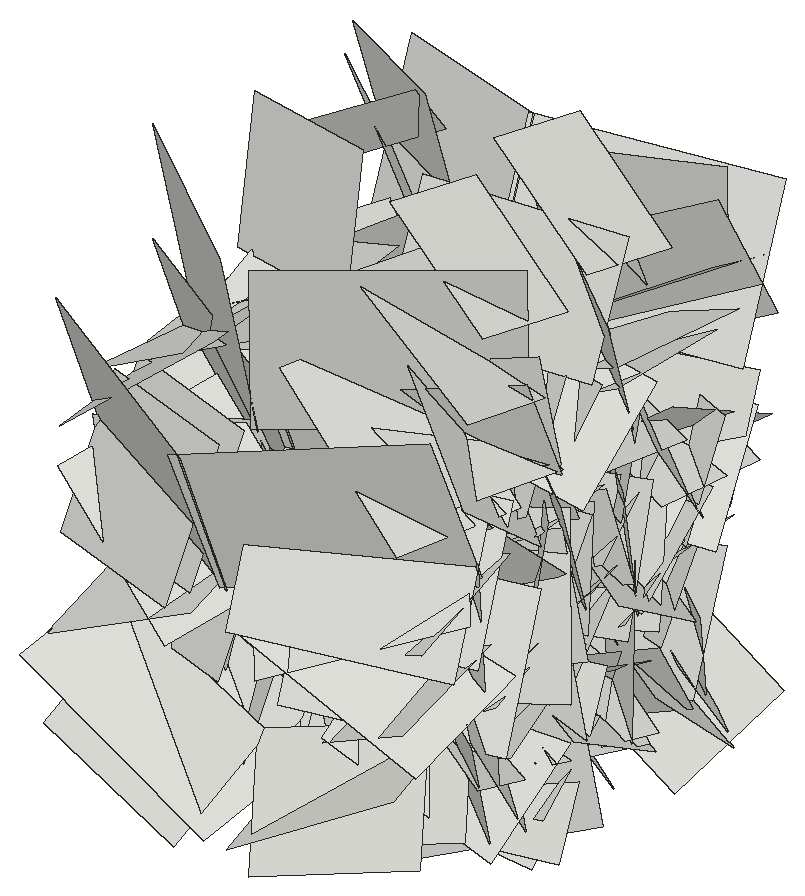
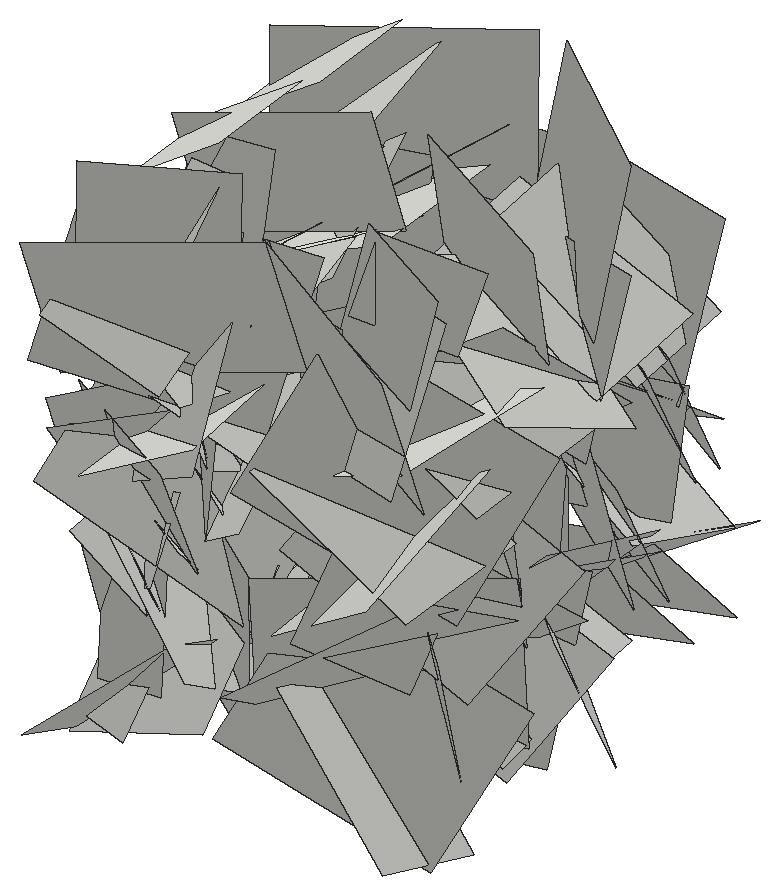
# SketchUp Ruby script. Lengths in inches.
U = 1.inch
M = Sketchup.active_model
def pt(a) = Geom::Point3d.new(a.map { |v| v * U })
def face(e, loops, mat)
  f = e.add_face(loops[0].map { |a| pt(a) })
  loops[1..].each { |l| e.add_face(l.map { |a| pt(a) }).erase! }
  f.material = f.back_material = mat if mat
  f
end
# faces: each face lists its corners as indices into pts; further lists are holes
def faces(e, pts, list, mat = nil) = list.each { |f| face(e, (f[0].is_a?(Array) ? f : [f]).map { |l| l.map { |i| pts[i] } }, mat) }
# xy, xz, yz: faces in a plane at the given z, y or x. An outline is a flat list of corners, or four numbers for a rectangle; further outlines are holes
def ring(l) = l.size == 4 ? [[l[0], l[1]], [l[2], l[1]], [l[2], l[3]], [l[0], l[3]]] : l.each_slice(2).to_a
def flat(e, list, mat, &to3) = list.each { |f| face(e, (f[0].is_a?(Array) ? f : [f]).map { |l| ring(l).map { |u, v| to3.(u, v) } }, mat) }
def xy(e, z, list, mat = nil) = flat(e, list, mat) { |x, y| [x, y, z] }
def xz(e, y, list, mat = nil) = flat(e, list, mat) { |x, z| [x, y, z] }
def yz(e, x, list, mat = nil) = flat(e, list, mat) { |y, z| [x, y, z] }
def lines(e, pts, list) = list.each { |a, b| e.add_line(pt(pts[a]), pt(pts[b])) }
# prism: a flat outline (further loops are holes) pulled along v
def prism(e, loops, v, mat = nil)
  f = face(e, loops, mat); d = Geom::Vector3d.new(v.map { |x| x * U })
  f.pushpull(f.normal.samedirection?(d) ? d.length : -d.length)
end
def box(e, o, s, mat = nil) = prism(e, [[o, [o[0] + s[0], o[1], o[2]], [o[0] + s[0], o[1] + s[1], o[2]], [o[0], o[1] + s[1], o[2]]]], [0, 0, s[2]], mat)
def at(x, y, z, deg = 0) = Geom::Transformation.translation(pt([x, y, z])) * Geom::Transformation.rotation(ORIGIN, Z_AXIS, deg.degrees)
def axes(o, x, y, z) = Geom::Transformation.new([*x, 0, *y, 0, *z, 0, *pt(o).to_a, 1])
def part(name) = M.definitions.add(name)
# library, detail: a bought-in or finely detailed component or shape, given as its bounding box
def library(name, o, s) = part(name).tap { |d| box(d.entities, o, s) }
def detail(e, o, s) = box(e.add_group.entities, o, s)
def put(e, d, t, mat = nil) = e.add_instance(d, t).tap { |i| i.material = mat if mat }
def group(e, t, mat = nil) = e.add_group.tap { |g| g.transformation = t; g.material = mat if mat }.entities
root = M.entities
c1 = part("Component\#6")
p = [[0.01,0,0],[0,3.24,4.54],[4.32,3.24,4.54],[4.33,0,0]]
faces(c1.entities,p,[[0,1,2,3]])
put(root,c1,axes([400.91,124,36.29],[-0.02149,0.52903,-1.24729],[0.2007,-1.23408,-0.5265],[1.42204,0.18216,0.05546]))
put(root,c1,axes([414.68,124,36.29],[0.02149,0.52903,-1.24729],[-0.2007,-1.23408,-0.5265],[-1.42204,0.18216,0.05546]))
put(root,c1,axes([400.85,123.49,22.43],[0.36857,0.54861,0.76203],[0.54406,0.56941,-0.64413],[0.83345,-0.61431,0.08349]))
put(root,c1,axes([414.74,123.49,22.43],[-0.36857,0.54861,0.76203],[-0.54406,0.56941,-0.64413],[-0.83345,-0.61431,0.08349]))
put(root,c1,axes([400.91,126.73,32.74],[-0.07983,-0.47542,-1.06148],[0.1788,-1.05692,0.46141],[1.21984,0.1238,-0.1371]))
put(root,c1,axes([414.68,126.73,32.74],[0.07983,-0.47542,-1.06148],[-0.1788,-1.05692,0.46141],[-1.21984,0.1238,-0.1371]))
put(root,c1,axes([400.91,122.33,25.2],[0.14417,1.26196,0.33106],[0.05821,0.32703,-1.26913],[1.38172,-0.14545,0.01892]))
put(root,c1,axes([414.68,122.33,25.2],[-0.14417,1.26196,0.33106],[-0.05821,0.32703,-1.26913],[-1.38172,-0.14545,0.01892]))
put(root,c1,axes([400.91,127.85,32.74],[-0.07983,-0.47542,-1.06148],[0.1788,-1.05692,0.46141],[1.21984,0.1238,-0.1371]))
put(root,c1,axes([414.68,127.85,32.74],[0.07983,-0.47542,-1.06148],[-0.1788,-1.05692,0.46141],[-1.21984,0.1238,-0.1371]))
put(root,c1,axes([400.91,128.39,27.01],[0.01413,-1.13969,-0.35832],[0.11214,-0.35581,1.13564],[1.2614,0.04439,-0.09695]))
put(root,c1,axes([414.68,128.39,27.01],[-0.01413,-1.13969,-0.35832],[-0.11214,-0.35581,1.13564],[-1.2614,0.04439,-0.09695]))
put(root,c1,axes([400.2,124.93,30.08],[0.69154,0.83647,0.57299],[0.50453,0.34895,-1.05134],[0.94895,-0.79509,0.14141]))
put(root,c1,axes([415.4,124.93,30.08],[-0.69154,0.83647,0.57299],[-0.50453,0.34895,-1.05134],[-0.94895,-0.79509,0.14141]))
put(root,c1,axes([410.71,128.06,26.23],[-0.10092,-0.80547,-0.37503],[-0.00485,-0.37672,0.81027],[0.94179,-0.08825,-0.03602]))
put(root,c1,axes([400.91,128.2,32.33],[0.15852,-1.12421,0.05612],[-0.12401,0.04078,1.12872],[1.18668,0.15444,0.11046]))
put(root,c1,axes([414.68,128.2,32.33],[-0.15852,-1.12421,0.05612],[0.12401,0.04078,1.12872],[-1.18668,0.15444,0.11046]))
put(root,c1,axes([400.85,125.55,22.43],[0.36857,0.54861,0.76203],[0.54406,0.56941,-0.64413],[0.83345,-0.61431,0.08349]))
put(root,c1,axes([414.74,125.55,22.43],[-0.36857,0.54861,0.76203],[-0.54406,0.56941,-0.64413],[-0.83345,-0.61431,0.08349]))
put(root,c1,axes([410.71,129.13,29.07],[-0.11411,-0.79222,-0.47459],[-0.01099,-0.47673,0.79815],[0.97884,-0.0977,-0.04636]))
put(root,c1,axes([400.91,128.47,40.0625],[0.15368,0.21217,-1.35934],[-0.08132,-1.3635,-0.221],[1.45608,-0.09854,0.13113]))
put(root,c1,axes([414.68,128.47,40.0625],[-0.15368,0.21217,-1.35934],[0.08132,-1.3635,-0.221],[-1.45608,-0.09854,0.13113]))
put(root,c1,axes([400.91,129.14,29.25],[-0.07983,-0.47542,-1.06148],[0.1788,-1.05692,0.46141],[1.21984,0.1238,-0.1371]))
put(root,c1,axes([414.68,129.14,29.25],[0.07983,-0.47542,-1.06148],[-0.1788,-1.05692,0.46141],[-1.21984,0.1238,-0.1371]))
put(root,c1,axes([414.68,126.77,21.87],[0.10992,-0.34124,0.92241],[-0.05569,0.92428,0.34784],[-1.04103,-0.08548,0.07879]))
put(root,c1,axes([414.68,129.34,35.47],[0.09463,-0.94647,0.23979],[0.00571,0.24126,0.95028],[-1.03494,-0.08521,0.02717]))
put(root,c1,axes([414.68,130.61,23.63],[0.04049,-0.92661,-0.53015],[0.18829,-0.51758,0.91743],[-1.11583,-0.12096,0.13557]))
put(root,c1,axes([400.91,126.5625,26.98],[-0.04661,-0.13743,1.04442],[0.16266,1.03335,0.14244],[1.10472,-0.15795,0.02309]))
put(root,c1,axes([414.68,126.5625,26.98],[0.04661,-0.13743,1.04442],[-0.16266,1.03335,0.14244],[-1.10472,-0.15795,0.02309]))
put(root,c1,axes([410.71,128.14,26.625],[-0.13018,-0.67547,0.62862],[-0.07474,0.63918,0.67304],[0.97523,-0.04118,0.13549]))
put(root,c1,axes([400.91,130.48,31.34],[-0.20009,-0.24055,-1.32848],[-0.01815,-1.34087,0.24522],[1.43098,-0.05064,-0.18264]))
put(root,c1,axes([414.68,130.48,31.34],[0.20009,-0.24055,-1.32848],[0.01815,-1.34087,0.24522],[-1.43098,-0.05064,-0.18264]))
put(root,c1,axes([410.71,126.29,27.49],[-0.18614,0.86586,-0.34095],[-0.04817,-0.35453,-0.87695],[0.98523,0.14625,-0.10729]))
put(root,c1,axes([400.91,130.13,32.75],[0.05656,-1.14018,0.16245],[0.17438,0.16851,1.12862],[1.20828,0.02906,-0.17049]))
put(root,c1,axes([414.68,130.13,32.75],[-0.05656,-1.14018,0.16245],[-0.17438,0.16851,1.12862],[-1.20828,0.02906,-0.17049]))
put(root,c1,axes([400.91,128.45,36.29],[-0.02149,0.52903,-1.24729],[0.2007,-1.23408,-0.5265],[1.42204,0.18216,0.05546]))
put(root,c1,axes([414.68,128.45,36.29],[0.02149,0.52903,-1.24729],[-0.2007,-1.23408,-0.5265],[-1.42204,0.18216,0.05546]))
put(root,c1,axes([414.68,129.02,36.97],[0.03047,0.19902,-0.90037],[-0.05941,-0.89877,-0.20045],[-0.97562,0.06094,-0.01591]))
put(root,c1,axes([414.68,130.54,26.21],[0.16316,0.13144,-1.2549],[0.21583,-1.25022,-0.10597],[-1.31994,-0.18819,-0.17245]))
put(root,c1,axes([414.68,129.15,30.625],[0.089,-0.93417,0.70597],[0.20388,0.70917,0.91554],[-1.22433,0.05019,0.20378]))
put(root,c1,axes([400.91,132.16,25.41],[-0.07094,-0.60211,-1.2376],[-0.1162,-1.23279,0.6057],[1.45423,-0.12788,-0.01197]))
put(root,c1,axes([414.68,132.16,25.41],[0.07094,-0.60211,-1.2376],[0.1162,-1.23279,0.6057],[-1.45423,-0.12788,-0.01197]))
put(root,c1,axes([414.68,130.09,30.86],[0.13772,0.10296,-1.023],[0.01142,-1.03121,-0.10242],[-1.08979,0.0022,-0.13035]))
put(root,c1,axes([414.68,130.39,37.85],[-0.05885,-0.83818,0.13983],[0.03078,0.13818,0.83979],[-0.90022,0.05952,0.01957]))
put(root,c1,axes([414.68,128.44,21.53],[0.07533,-0.68545,1.00594],[0.30491,0.98857,0.65329],[-1.25377,0.19923,0.21932]))
put(root,c1,axes([414.68,131.26,22.93],[-0.10206,-0.4663,-0.72841],[-0.02316,-0.73136,0.47108],[-0.91647,0.07041,0.06921]))
put(root,c1,axes([400.91,131.47,30.67],[0.19347,-0.24403,-0.96391],[-0.05093,-0.98104,0.23927],[1.05275,-0.00261,0.18872]))
put(root,c1,axes([414.68,131.47,30.67],[-0.19347,-0.24403,-0.96391],[0.05093,-0.98104,0.23927],[-1.05275,-0.00261,0.18872]))
put(root,c1,axes([400.91,131.58,31.0625],[0.07279,0.01987,-1.05868],[-0.10279,-1.05633,-0.02611],[1.11768,-0.09844,0.06655]))
put(root,c1,axes([414.68,131.58,31.0625],[-0.07279,0.01987,-1.05868],[0.10279,-1.05633,-0.02611],[-1.11768,-0.09844,0.06655]))
put(root,c1,axes([400.91,131.52,23.18],[0.15485,-0.9106,-0.00305],[0.11373,0.01414,0.91588],[0.95852,0.14543,-0.10818]))
put(root,c1,axes([414.68,131.52,23.18],[-0.15485,-0.9106,-0.00305],[-0.11373,0.01414,0.91588],[-0.95852,0.14543,-0.10818]))
put(root,c1,axes([400.91,127.05,26.22],[0.14417,1.26196,0.33106],[0.05821,0.32703,-1.26913],[1.38172,-0.14545,0.01892]))
put(root,c1,axes([414.68,127.05,26.22],[-0.14417,1.26196,0.33106],[-0.05821,0.32703,-1.26913],[-1.38172,-0.14545,0.01892]))
put(root,c1,axes([414.68,127.73,24.28],[0.02979,0.75993,0.53946],[0.00151,0.53967,-0.7603],[-0.98786,0.02374,0.0151]))
put(root,c1,axes([400.91,127.1,26.99],[-0.01407,1.25738,0.35681],[-0.29384,0.346,-1.2296],[1.35392,0.08816,-0.26315]))
put(root,c1,axes([414.68,127.1,26.99],[0.01407,1.25738,0.35681],[0.29384,0.346,-1.2296],[-1.35392,0.08816,-0.26315]))
put(root,c1,axes([414.68,129.03,31.05],[-0.04043,0.74356,0.04678],[-0.07255,0.04314,-0.74161],[-0.78639,-0.04221,0.06601]))
put(root,c1,axes([400.91,134.48,33.76],[-0.26334,-1.11466,-0.41014],[0.1173,-0.43892,1.12584],[1.25351,-0.19309,-0.19152]))
put(root,c1,axes([414.68,134.48,33.76],[0.26334,-1.11466,-0.41014],[-0.1173,-0.43892,1.12584],[-1.25351,-0.19309,-0.19152]))
put(root,c1,axes([410.71,133.52,31.89],[-0.15087,-0.04242,-1.05475],[-0.23169,-1.04005,0.07132],[1.09469,-0.22597,-0.13027]))
put(root,c1,axes([414.68,129.22,21.54],[0.01805,0.58513,0.55019],[-0.06792,0.54955,-0.58247],[-0.84865,-0.03153,0.05832]))
put(root,c1,axes([410.71,129.75,30.06],[0.01937,0.49926,0.36665],[0.0577,0.36409,-0.4985],[0.65405,-0.04691,0.03312]))
put(root,c1,axes([400.91,133.17,39.1],[0.0845,-0.28698,-1.03421],[0.22383,-1.0126,0.29726],[1.11545,0.22493,0.0187]))
put(root,c1,axes([414.68,133.17,39.1],[-0.0845,-0.28698,-1.03421],[-0.22383,-1.0126,0.29726],[-1.11545,0.22493,0.0187]))
put(root,c1,axes([400.91,128.43,31.91],[0.33386,1.00192,0.91989],[0.02581,0.93993,-1.03208],[1.44154,-0.24887,-0.19457]))
put(root,c1,axes([414.68,128.43,31.91],[-0.33386,1.00192,0.91989],[-0.02581,0.93993,-1.03208],[-1.44154,-0.24887,-0.19457]))
put(root,c1,axes([410.71,130.92,26.67],[-0.06799,-0.20959,0.7931],[0.02884,0.79454,0.21217],[0.86907,-0.04277,0.05501]))
put(root,c1,axes([414.68,131.21,27.63],[0.2234,-0.54463,1.08834],[0.02633,1.10624,0.54877],[-1.28976,-0.07175,0.19972]))
put(root,c1,axes([400.91,134.27,30.6],[0.0256,-0.22889,-1.14247],[0.00761,-1.14266,0.22909],[1.23506,0.01178,0.02227]))
put(root,c1,axes([414.68,134.27,30.6],[-0.0256,-0.22889,-1.14247],[-0.00761,-1.14266,0.22909],[-1.23506,0.01178,0.02227]))
put(root,c1,axes([410.71,134.18,33.55],[-0.07538,-0.44425,-0.62436],[0.04133,-0.62833,0.44263],[0.8112,-0.00926,-0.08057]))
put(root,c1,axes([414.68,134.17,21.91],[0.00769,-1.04417,0.30366],[0.13881,0.30229,1.03635],[-1.14428,0.02965,0.12776]))
put(root,c1,axes([400.91,134.58,22.11],[0.07114,-1.22092,0.271],[-0.02912,0.26988,1.2227],[1.32535,0.07146,0.01232]))
put(root,c1,axes([414.68,134.58,22.11],[-0.07114,-1.22092,0.271],[0.02912,0.26988,1.2227],[-1.32535,0.07146,0.01232]))
put(root,c1,axes([400.91,134.42,21.5625],[-0.1234,-1.02964,0.56694],[0.11588,0.55776,1.03542],[1.24053,-0.15452,-0.04032]))
put(root,c1,axes([414.68,134.42,21.5625],[0.1234,-1.02964,0.56694],[-0.11588,0.55776,1.03542],[-1.24053,-0.15452,-0.04032]))
put(root,c1,axes([400.91,132.49,21.15],[0.19066,-0.73145,1.17679],[0.11238,1.19045,0.72374],[1.46442,0.00387,-0.20876]))
put(root,c1,axes([414.68,132.49,21.15],[-0.19066,-0.73145,1.17679],[-0.11238,1.19045,0.72374],[-1.46442,0.00387,-0.20876]))
put(root,c1,axes([410.71,134.6875,22.2],[-0.10426,-0.66856,0.17597],[0.06243,0.169,0.67497],[0.73015,-0.10992,-0.03258]))
put(root,c1,axes([410.71,131.06,25.92],[-0.11704,0.23417,0.88186],[-0.10525,0.87993,-0.24609],[0.96142,0.12483,0.08041]))
put(root,c1,axes([400.91,130.54,25.39],[0.14552,0.87979,0.74939],[0.0105,0.75374,-0.8867],[1.22498,-0.11098,-0.08143]))
put(root,c1,axes([414.68,130.54,25.39],[-0.14552,0.87979,0.74939],[-0.0105,0.75374,-0.8867],[-1.22498,-0.11098,-0.08143]))
put(root,c1,axes([400.91,135.84,31.22],[-0.16391,-1.12855,0.28901],[0.13375,0.27361,1.13591],[1.2276,-0.1805,-0.08517]))
put(root,c1,axes([414.68,135.84,31.22],[0.16391,-1.12855,0.28901],[-0.13375,0.27361,1.13591],[-1.2276,-0.1805,-0.08517]))
put(root,c1,axes([414.68,135.18,37.85],[-0.05885,-0.83818,0.13983],[0.03078,0.13818,0.83979],[-0.90022,0.05952,0.01957]))
put(root,c1,axes([414.68,133.37,32.625],[0.2234,-0.54463,1.08834],[0.02633,1.10624,0.54877],[-1.28976,-0.07175,0.19972]))
put(root,c1,axes([414.68,131.97,28.78],[-0.10091,0.74431,0.53228],[0.01265,0.53611,-0.74754],[-0.96987,-0.07045,-0.06513]))
put(root,c1,axes([404.88,136.41,29.65],[0.07813,-0.63244,-0.26103],[0.10098,-0.25049,0.63382],[-0.71818,-0.10402,0.06072]))
put(root,c1,axes([410.71,136.41,29.65],[-0.07813,-0.63244,-0.26103],[-0.10098,-0.25049,0.63382],[0.71818,-0.10402,0.06072]))
put(root,c1,axes([414.68,134.54,24.9375],[-0.02484,0.40022,-0.64969],[-0.07983,-0.64803,-0.39648],[-0.8049,0.05192,0.05937]))
put(root,c1,axes([400.91,136.25,25.03],[-0.1909,-1.05424,0.65515],[0.04228,0.65676,1.06778],[1.31502,-0.17416,0.06077]))
put(root,c1,axes([414.68,136.25,25.03],[0.1909,-1.05424,0.65515],[-0.04228,0.65676,1.06778],[-1.31502,-0.17416,0.06077]))
put(root,c1,axes([400.91,132.63,34.3],[0.186,1.33026,-0.17859],[0.24164,-0.20703,-1.31812],[1.40205,-0.1408,0.25087]))
put(root,c1,axes([414.68,132.63,34.3],[-0.186,1.33026,-0.17859],[-0.24164,-0.20703,-1.31812],[-1.40205,-0.1408,0.25087]))
put(root,c1,axes([414.68,132.79,29.8],[-0.04873,0.29435,0.84438],[0.1159,0.841,-0.28722],[-0.94075,0.08836,-0.07912]))
put(root,c1,axes([400.91,137.68,26.93],[0.04018,-0.30696,-1.06119],[-0.15368,-1.05402,0.2997],[1.16085,-0.12891,0.07641]))
put(root,c1,axes([414.68,137.68,26.93],[-0.04018,-0.30696,-1.06119],[0.15368,-1.05402,0.2997],[-1.16085,-0.12891,0.07641]))
put(root,c1,axes([414.68,133.57,26.39],[0.0097,-0.16576,1.00827],[0.11893,1.00238,0.16377],[-1.07657,0.10924,0.02717]))
put(root,c1,axes([410.71,135.55,39.48],[0.03347,0.37514,-0.47819],[-0.05412,-0.47551,-0.37641],[0.64197,-0.05964,-0.0068]))
put(root,c1,axes([404.88,135.55,39.48],[-0.03347,0.37514,-0.47819],[0.05412,-0.47551,-0.37641],[-0.64197,-0.05964,-0.0068]))
put(root,c1,axes([414.68,132.63,35],[0.22269,1.01925,0.0867],[-0.15354,0.11726,-1.02752],[-1.07338,0.19468,0.16497]))
put(root,c1,axes([400.91,133.32,22.11],[0.03082,0.0656,1.39488],[-0.001,1.39518,-0.0656],[1.48021,-0.00042,-0.02909]))
put(root,c1,axes([414.68,133.32,22.11],[-0.03082,0.0656,1.39488],[0.001,1.39518,-0.0656],[-1.48021,-0.00042,-0.02909]))
put(root,c1,axes([414.68,133.77,26.39],[0.09062,0.64279,0.71838],[-0.13606,0.72237,-0.63108],[-1.01272,-0.03954,0.14907]))
put(root,c1,axes([414.68,139.12,30.95],[0.15428,-0.64193,-0.79007],[-0.04846,-0.80142,0.64273],[-1.07797,-0.05585,-0.14197]))
put(root,c1,axes([414.68,134.64,27.51],[-0.11331,0.92563,-0.03565],[0.09128,-0.0258,-0.92812],[-0.97764,-0.10969,-0.08252]))
put(root,c1,axes([400.91,135.17,32.61],[0.12448,1.21649,-0.63228],[-0.14654,-0.62086,-1.22019],[1.44585,-0.16766,-0.06923]))
put(root,c1,axes([414.68,135.17,32.61],[-0.12448,1.21649,-0.63228],[0.14654,-0.62086,-1.22019],[-1.44585,-0.16766,-0.06923]))
put(root,c1,axes([400.91,136.8125,27.97],[-0.23976,-0.84366,1.03424],[-0.08712,1.0558,0.84327],[1.41209,-0.07811,0.22763]))
put(root,c1,axes([414.68,136.8125,27.97],[0.23976,-0.84366,1.03424],[0.08712,1.0558,0.84327],[-1.41209,-0.07811,0.22763]))
put(root,c1,axes([400.91,132.97,26.35],[0.04012,1.17129,0.65858],[-0.12839,0.65914,-1.16531],[1.41857,0.02653,-0.1241]))
put(root,c1,axes([414.68,132.97,26.35],[-0.04012,1.17129,0.65858],[0.12839,0.65914,-1.16531],[-1.41857,0.02653,-0.1241]))
put(root,c1,axes([400.91,137.29,38.52],[-0.00887,0.62519,-1.13199],[-0.07674,-1.13046,-0.62381],[1.3686,-0.05933,-0.04231]))
put(root,c1,axes([414.68,137.29,38.52],[0.00887,0.62519,-1.13199],[0.07674,-1.13046,-0.62381],[-1.3686,-0.05933,-0.04231]))
put(root,c1,axes([410.71,134.33,29.51],[-0.0444,0.3698,0.86525],[-0.11423,0.85852,-0.37214],[0.99086,0.11554,-0.00413]))
put(root,c1,axes([400.91,139.23,29.07],[-0.06497,-1.13195,0.1646],[0.10003,0.15928,1.13044],[1.20835,-0.07404,-0.08473]))
put(root,c1,axes([414.68,139.23,29.07],[0.06497,-1.13195,0.1646],[-0.10003,0.15928,1.13044],[-1.20835,-0.07404,-0.08473]))
put(root,c1,axes([400.91,137.68,39.44],[0.12024,0.16456,-0.83242],[0.12638,-0.83458,-0.14874],[0.89051,0.09622,0.13351]))
put(root,c1,axes([414.68,137.68,39.44],[-0.12024,0.16456,-0.83242],[-0.12638,-0.83458,-0.14874],[-0.89051,0.09622,0.13351]))
put(root,c1,axes([400.91,138.04,20.07],[-0.12016,-0.9858,0.86253],[0.12902,0.85408,0.99214],[1.38246,-0.16539,-0.01763]))
put(root,c1,axes([414.68,138.04,20.07],[0.12016,-0.9858,0.86253],[-0.12902,0.85408,0.99214],[-1.38246,-0.16539,-0.01763]))
put(root,c1,axes([410.71,139.13,26.61],[-0.02912,-0.4172,-0.72752],[-0.02466,-0.72725,0.41792],[0.88863,-0.03385,-0.01224]))
put(root,c1,axes([400.91,140.34,20.98],[0.05969,-1.08852,-0.33352],[-0.17093,-0.33819,1.07653],[1.19461,0.00599,0.1707]))
put(root,c1,axes([414.68,140.34,20.98],[-0.05969,-1.08852,-0.33352],[0.17093,-0.33819,1.07653],[-1.19461,0.00599,0.1707]))
put(root,c1,axes([410.71,137.74,29.49],[-0.05063,0.39266,-0.56355],[-0.15447,-0.55784,-0.37633],[0.71149,-0.09317,-0.12181]))
put(root,c1,axes([404.88,137.74,29.49],[0.05063,0.39266,-0.56355],[0.15447,-0.55784,-0.37633],[-0.71149,-0.09317,-0.12181]))
put(root,c1,axes([414.68,135.78,27.7],[0.08438,0.31612,0.89331],[-0.15155,0.8902,-0.30228],[-0.99295,-0.109,0.12205]))
put(root,c1,axes([400.91,140.4,37.84],[-0.00777,-0.46206,-1.23937],[0.21731,-1.22481,0.45542],[1.38512,0.18957,-0.0784]))
put(root,c1,axes([414.68,140.4,37.84],[0.00777,-0.46206,-1.23937],[-0.21731,-1.22481,0.45542],[-1.38512,0.18957,-0.0784]))
put(root,c1,axes([410.71,138.35,27.1],[-0.19626,0.31166,-0.79897],[0.02742,-0.81497,-0.3239],[0.90864,0.09191,-0.1628]))
put(root,c1,axes([414.68,137.01,36.4],[-0.10049,0.69541,-0.2411],[-0.01368,-0.24463,-0.7005],[-0.78006,-0.08529,0.04335]))
put(root,c1,axes([414.68,137.76,20.74],[-0.07875,-0.43706,0.66864],[0.02301,0.67018,0.44047],[-0.84643,0.05888,-0.05024]))
